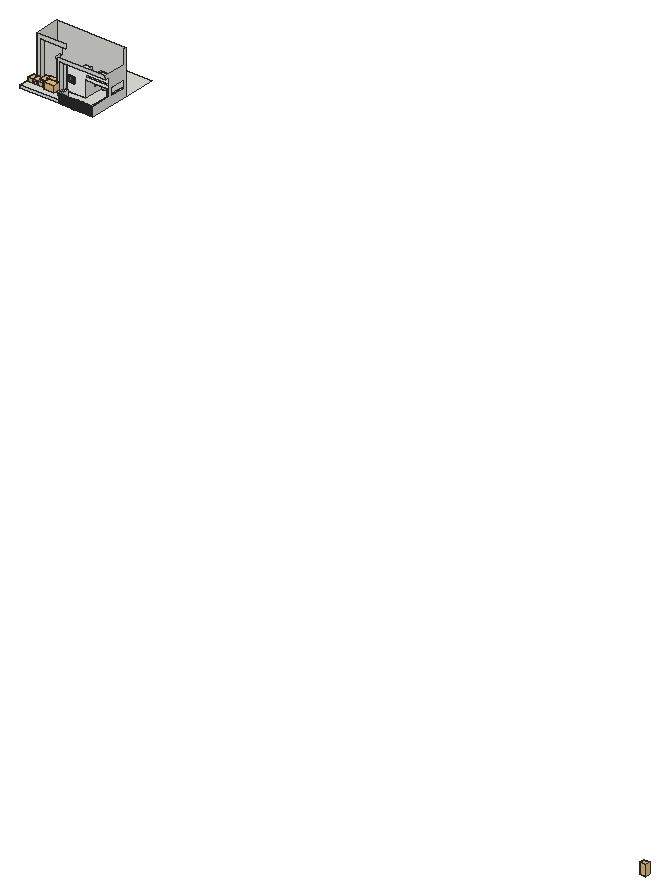
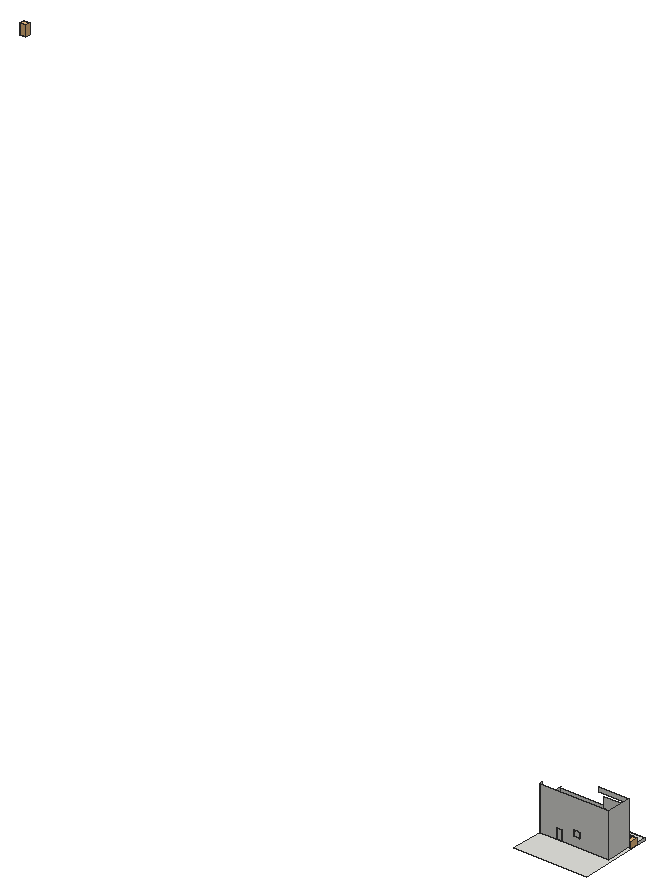
# SketchUp Ruby script. Lengths in inches.
U = 1.inch
M = Sketchup.active_model
def pt(a) = Geom::Point3d.new(a.map { |v| v * U })
def face(e, loops, mat)
  f = e.add_face(loops[0].map { |a| pt(a) })
  loops[1..].each { |l| e.add_face(l.map { |a| pt(a) }).erase! }
  f.material = f.back_material = mat if mat
  f
end
# faces: each face lists its corners as indices into pts; further lists are holes
def faces(e, pts, list, mat = nil) = list.each { |f| face(e, (f[0].is_a?(Array) ? f : [f]).map { |l| l.map { |i| pts[i] } }, mat) }
# xy, xz, yz: faces in a plane at the given z, y or x. An outline is a flat list of corners, or four numbers for a rectangle; further outlines are holes
def ring(l) = l.size == 4 ? [[l[0], l[1]], [l[2], l[1]], [l[2], l[3]], [l[0], l[3]]] : l.each_slice(2).to_a
def flat(e, list, mat, &to3) = list.each { |f| face(e, (f[0].is_a?(Array) ? f : [f]).map { |l| ring(l).map { |u, v| to3.(u, v) } }, mat) }
def xy(e, z, list, mat = nil) = flat(e, list, mat) { |x, y| [x, y, z] }
def xz(e, y, list, mat = nil) = flat(e, list, mat) { |x, z| [x, y, z] }
def yz(e, x, list, mat = nil) = flat(e, list, mat) { |y, z| [x, y, z] }
def lines(e, pts, list) = list.each { |a, b| e.add_line(pt(pts[a]), pt(pts[b])) }
# prism: a flat outline (further loops are holes) pulled along v
def prism(e, loops, v, mat = nil)
  f = face(e, loops, mat); d = Geom::Vector3d.new(v.map { |x| x * U })
  f.pushpull(f.normal.samedirection?(d) ? d.length : -d.length)
end
def box(e, o, s, mat = nil) = prism(e, [[o, [o[0] + s[0], o[1], o[2]], [o[0] + s[0], o[1] + s[1], o[2]], [o[0], o[1] + s[1], o[2]]]], [0, 0, s[2]], mat)
def at(x, y, z, deg = 0) = Geom::Transformation.translation(pt([x, y, z])) * Geom::Transformation.rotation(ORIGIN, Z_AXIS, deg.degrees)
def axes(o, x, y, z) = Geom::Transformation.new([*x, 0, *y, 0, *z, 0, *pt(o).to_a, 1])
def part(name) = M.definitions.add(name)
# library, detail: a bought-in or finely detailed component or shape, given as its bounding box
def library(name, o, s) = part(name).tap { |d| box(d.entities, o, s) }
def detail(e, o, s) = box(e.add_group.entities, o, s)
def put(e, d, t, mat = nil) = e.add_instance(d, t).tap { |i| i.material = mat if mat }
def group(e, t, mat = nil) = e.add_group.tap { |g| g.transformation = t; g.material = mat if mat }.entities
root = M.entities
M.materials.add("[0131_Silver]").color = [192, 192, 192]
M.materials.add("[Color M00]").color = [255, 255, 255]
M.materials.add("[Translucent Glass Gray]").color = [128, 128, 128]
M.materials["[Translucent Glass Gray]"].alpha = 0.5
M.materials.add("[Wood Floor]").color = [155, 105, 61]
M.materials.add("efeu2").color = [43, 57, 29]
c1 = library("Broadleaf plant",[0,0,0],[149.19,166.1,98.1875])
c2 = library("N_Plant_4",[-12.12,-0.17,0],[15.33,15.33,4.43])
c3 = library("door by lz",[5.91,-4.92,0],[35.43,6.61,78.74])
c4 = part("Gate frame")
xy(c4.entities,0,[[[0,0,66,72],[3,3,48,69],[51,3,63,69]]])
xy(c4.entities,0.5,[[3,3,48,69]])
xy(c4.entities,1.5,[[3,3,48,11.25],[3,11.25,48,19.5],[3,19.5,48,27.75],[3,27.75,48,36],[3,36,48,44.25],
  [3,44.25,48,52.5],[3,52.5,48,60.75],[3,60.75,48,69]])
xy(c4.entities,2,[[[0,0,66,72],[3,3,48,69],[51,3,63,69]]])
xz(c4.entities,0,[[0,0,51,2],[51,0,66,2]])
xz(c4.entities,3,[[3,0,27,0.5],[27,0,48,0.5],[51,0,63,2],[3,1.5,48,2]])
xz(c4.entities,69,[[3,0,48,0.5],[51,0,63,2],[3,1.5,48,2]])
xz(c4.entities,72,[[0,0,66,2]])
yz(c4.entities,0,[[0,0,72,2]])
yz(c4.entities,3,[[3,0,69,0.5],[3,1.5,69,2]])
yz(c4.entities,48,[[3,0,69,0.5],[3,1.5,69,2]])
yz(c4.entities,51,[[3,0,69,2]])
yz(c4.entities,63,[[3,0,69,2]])
yz(c4.entities,66,[[0,0,72,2]])
c5 = part("Horizontal gate bar")
box(c5.entities,[0,0,0],[12,1,1])
c6 = part("Slatted gate insert")
put(c6.entities,c5,at(3,0.5,22.5))
put(c6.entities,c5,at(3,0.5,26.5))
put(c6.entities,c5,at(3,0.5,28.5))
put(c6.entities,c5,at(3,0.5,4.5))
put(c6.entities,c5,at(3,0.5,2.5))
put(c6.entities,c5,at(3,0.5,54.5))
put(c6.entities,c5,at(3,0.5,56.5))
put(c6.entities,c5,at(3,0.5,24.5))
put(c6.entities,c5,at(3,0.5,20.5))
put(c6.entities,c5,at(3,0.5,34.5))
put(c6.entities,c5,at(3,0.5,6.5))
put(c6.entities,c5,at(3,0.5,42.5))
put(c6.entities,c5,at(3,0.5,0.5))
put(c6.entities,c5,at(3,0.5,10.5))
put(c6.entities,c5,at(3,0.5,16.5))
put(c6.entities,c5,at(3,0.5,18.5))
put(c6.entities,c5,at(3,0.5,58.5))
put(c6.entities,c5,at(3,0.5,40.5))
put(c6.entities,c5,at(3,0.5,60.5))
put(c6.entities,c5,at(3,0.5,36.5))
put(c6.entities,c5,at(3,0.5,38.5))
put(c6.entities,c5,at(3,0.5,32.5))
put(c6.entities,c5,at(3,0.5,8.5))
put(c6.entities,c5,at(3,0.5,64.5))
put(c6.entities,c5,at(3,0.5,12.5))
put(c6.entities,c5,at(3,0.5,44.5))
put(c6.entities,c5,at(3,0.5,46.5))
put(c6.entities,c5,at(3,0.5,52.5))
put(c6.entities,c5,at(3,0.5,48.5))
put(c6.entities,c5,at(3,0.5,50.5))
put(c6.entities,c5,at(3,0.5,62.5))
put(c6.entities,c5,at(3,0.5,14.5))
put(c6.entities,c5,at(3,0.5,30.5))
c7 = part("Gate panel slat")
xy(c7.entities,0.25,[[0.25,0,44.75,0.15]])
xy(c7.entities,8,[[0.25,0,44.75,0.15]])
xz(c7.entities,0,[[0.25,0.25,44.75,8]])
xz(c7.entities,0.15,[[[0,0,45,8.25],[0.25,0.25,44.75,8]]])
yz(c7.entities,0.25,[[0,0.25,0.15,8]])
yz(c7.entities,44.75,[[0,0.25,0.15,8]])
p = [[0,0.15,0],[0.25,0,0.25],[44.75,0,0.25],[45,0.15,0],[0,0.15,8.25],[0.25,0,8],
  [44.75,0,8],[45,0.15,8.25]]
faces(c7.entities,p,[[0,1,2,3],[4,5,1,0],[3,2,6,7],[5,4,7,6]])
c8 = part("Gate infill panel")
put(c8.entities,c7,at(0,0,24.75))
put(c8.entities,c7,at(0,0,57.75))
put(c8.entities,c7,at(0,0,49.5))
put(c8.entities,c7,at(0,0,41.25))
put(c8.entities,c7,at(0,0,33))
put(c8.entities,c7,axes([0,1.3,49.5],[1,0,0],[0,-1,0],[0,0,1]))
put(c8.entities,c7,at(0,0,16.5))
put(c8.entities,c7,at(0,0,8.25))
put(c8.entities,c7,axes([0,1.3,24.75],[1,0,0],[0,-1,0],[0,0,1]))
put(c8.entities,c7,at(0,0,0))
put(c8.entities,c7,axes([0,1.3,57.75],[1,0,0],[0,-1,0],[0,0,1]))
put(c8.entities,c7,axes([0,1.3,41.25],[1,0,0],[0,-1,0],[0,0,1]))
put(c8.entities,c7,axes([0,1.3,33],[1,0,0],[0,-1,0],[0,0,1]))
put(c8.entities,c7,axes([0,1.3,16.5],[1,0,0],[0,-1,0],[0,0,1]))
put(c8.entities,c7,axes([0,1.3,8.25],[1,0,0],[0,-1,0],[0,0,1]))
put(c8.entities,c7,axes([0,1.3,0],[1,0,0],[0,-1,0],[0,0,1]))
c9 = part("Entrance gate leaf")
put(c9.entities,c4,axes([0,2,0],[1,0,0],[0,0,1],[0,-1,0]),"[0131_Silver]")
put(c9.entities,c6,at(48,0,3),"[0131_Silver]")
put(c9.entities,c8,at(3,0.35,3))
c10 = part("Gate pull handle")
prism(c10.entities,[[[0.35,0,3.8],[0.35,0,3],[0.35,-1.5,3],[0.35,-1.5,51],[0.35,0,51],[0.35,0,50.2],[0.35,-1,50.2],[0.35,-1,3.8]]],[0.8,0,0])
c11 = part("gate1")
g1 = group(c11.entities,at(123.625,43.75,0))
put(g1,c9,at(0,1.5,0))
put(g1,c10,at(67.25,1.5,9),"[0131_Silver]")
put(g1,c10,at(63.75,1.5,9),"[0131_Silver]")
put(g1,c9,axes([132.5,1.5,0],[-1,0,0],[0,1,0],[0,0,1]))
c12 = part("window full")
xy(c12.entities,0,[[0,0,14.17,66.54]])
xy(c12.entities,2.26,[[12.2,2.26,14.17,64.28]],"[Wood Floor]")
xy(c12.entities,2.36,[[0,2.36,1.97,64.17]],"[Wood Floor]")
xy(c12.entities,3.74,[[11.42,3.74,12.2,32.875],[11.42,33.66,12.2,62.79]],"[Wood Floor]")
xy(c12.entities,3.9375,[[1.97,3.9375,2.76,32.77],[1.97,33.76,2.76,62.6]],"[Wood Floor]")
xy(c12.entities,4.18,[[2.76,4.18,7.09,32.09],[7.09,4.18,11.42,32.09],[2.76,34.45,7.09,62.35],[7.09,34.45,11.42,62.35]],"[Wood Floor]")
xy(c12.entities,69.83,[[2.76,4.18,7.09,32.09],[7.09,32.09,11.42,34.45],[2.76,34.45,7.09,62.35]])
xy(c12.entities,69.83,[[7.09,4.18,11.42,32.09],[7.09,34.45,11.42,62.35]],"[Wood Floor]")
xy(c12.entities,70.08,[[1.97,3.9375,2.76,32.77],[1.97,33.76,2.76,62.6]])
xy(c12.entities,70.27,[[11.42,32.875,12.2,33.66]])
xy(c12.entities,70.27,[[11.42,3.74,12.2,32.875],[11.42,33.66,12.2,62.79]],"[Wood Floor]")
xy(c12.entities,71.65,[[0,2.36,1.97,64.17]])
xy(c12.entities,71.76,[[12.2,2.26,14.17,64.28]],"[Wood Floor]")
xy(c12.entities,74.02,[[0,0,14.17,66.54]],"[Wood Floor]")
xz(c12.entities,0,[[0,0,14.17,74.02]],"[Wood Floor]")
xz(c12.entities,2.26,[[12.2,2.26,14.17,71.76]],"[Wood Floor]")
xz(c12.entities,2.36,[[0,2.36,1.97,71.65]],"[Wood Floor]")
xz(c12.entities,3.74,[[11.42,3.74,12.2,70.27]],"[Wood Floor]")
xz(c12.entities,3.9375,[[1.97,3.9375,2.76,70.08]],"[Wood Floor]")
xz(c12.entities,4.18,[[2.76,4.18,7.09,69.83],[7.09,4.18,11.42,69.83]],"[Wood Floor]")
xz(c12.entities,32.09,[[2.76,4.18,11.42,69.83]],"[Wood Floor]")
xz(c12.entities,32.77,[[1.97,3.9375,2.76,70.08]],"[Wood Floor]")
xz(c12.entities,32.875,[[11.42,3.74,12.2,70.27]],"[Wood Floor]")
xz(c12.entities,33.66,[[11.42,3.74,12.2,47.88],[11.42,47.88,12.2,70.27]],"[Wood Floor]")
xz(c12.entities,33.76,[[1.97,3.9375,2.76,70.08]],"[Wood Floor]")
xz(c12.entities,34.45,[[2.76,4.18,11.42,69.83]],"[Wood Floor]")
xz(c12.entities,62.35,[[2.76,4.18,7.09,69.83],[7.09,4.18,11.42,69.83]],"[Wood Floor]")
xz(c12.entities,62.6,[[1.97,3.9375,2.76,70.08]],"[Wood Floor]")
xz(c12.entities,62.79,[[11.42,3.74,12.2,70.27]],"[Wood Floor]")
xz(c12.entities,64.17,[[0,2.36,1.97,71.65]],"[Wood Floor]")
xz(c12.entities,64.28,[[12.2,2.26,14.17,71.76]],"[Wood Floor]")
xz(c12.entities,66.54,[[0,0,14.17,74.02]],"[Wood Floor]")
yz(c12.entities,0,[[[0,0,66.54,74.02],[2.36,2.36,64.17,71.65]]],"[Wood Floor]")
yz(c12.entities,1.97,[[[2.36,2.36,64.17,71.65],[33.76,3.9375,62.6,70.08],[3.9375,3.9375,32.77,70.08]]],"[Wood Floor]")
yz(c12.entities,2.76,[[32.77,3.9375,33.76,4.18],[32.77,4.18,33.76,69.83],[32.77,69.83,33.76,70.08]])
yz(c12.entities,2.76,[[[3.9375,3.9375,32.77,70.08],[4.18,4.18,32.09,69.83]],[[33.76,3.9375,62.6,70.08],[34.45,4.18,62.35,69.83]]],"[Wood Floor]")
yz(c12.entities,7.09,[[4.18,4.18,62.35,69.83]],"[Translucent Glass Gray]")
yz(c12.entities,11.42,[[32.875,69.83,33.66,70.27]])
yz(c12.entities,11.42,[[[3.74,3.74,32.875,70.27],[4.18,4.18,32.09,69.83]],[[33.66,3.74,62.79,70.27],[34.45,4.18,62.35,69.83]]],"[Wood Floor]")
yz(c12.entities,12.2,[[[2.26,2.26,64.28,71.76],[3.74,3.74,32.875,70.27],[33.66,3.74,62.79,70.27]]],"[Wood Floor]")
yz(c12.entities,14.17,[[[0,0,66.54,74.02],[2.26,2.26,64.28,71.76]]],"[Wood Floor]")
p = [[11.42,32.875,70.27],[11.42,32.875,70.28]]
lines(c12.entities,p,[[0,1]])
c13 = library("climbing plant",[8874.76,-5589.78,-33.625],[50.13,38.07,87.16])
c14 = part("ivyleaf_10")
p = [[0,0.5,-0.03],[-0.0625,2.02,-0.43],[-0.19,2.01,-0.46],[-0.54,1.05,-0.29],[-0.52,0.625,-0.18],[-0.83,0.76,-0.28],
  [-1.16,0.64,-0.33],[-1.15,0.33,-0.24],[-0.77,-0.39,0.02],[-0.3,-0.51,0.16],[0.04,-0.48,0.23],[-0.02,2.01,-0.4375],
  [-0.06,2.01,-0.43],[0.04,-0.49,0.23],[0.67,-0.49,0.14],[1.38,0.36,-0.2],[1.375,0.51,-0.24],[0.81,0.65,-0.19],
  [0.62,0.59,-0.15],[0.6,1.09,-0.28],[0.5,1.23,-0.31]]
faces(c14.entities,p,[[0,1,2,3,4,5,6,7,8,9,10],[11,12,0,13,14,15,16,17,18,19,20]],"efeu2")
xy(root,0,[[0,7.0625,315.8125,80.4375],[336.86,7.0625,583.09,7.0625,583.09,321.4375,460.26,321.4375,460.26,345.4375,412.26,345.4375,412.26,172.6875,255.63,172.6875,255.63,166.9375,222.91,166.9375,222.91,139.625,196.34,139.625,196.34,172.6875,63.85,172.6875,63.85,139.625,29.66,139.625,29.66,345.4375,600,345.4375,600,607.0625,0,607.0625,0,80.4375,315.8125,80.4375,315.8125,81.3125,336.86,81.3125],[583.09,7.0625,600,81.3125],[583.09,81.3125,600,172.6875],[29.66,139.625,29.66,345.4375,412.26,345.4375,412.26,172.6875,255.63,172.6875,255.63,166.9375,222.91,166.9375,222.91,139.625,196.34,139.625,196.34,172.6875,63.85,172.6875,63.85,139.625],
  [583.09,172.6875,583.09,321.4375,460.26,321.4375,460.26,345.4375,600,345.4375,600,172.6875]])
xy(root,23.375,[[0,7.0625,315.8125,80.4375]])
xy(root,65.15,[[583.09,0,600,7.0625]])
xy(root,65.68,[[315.8125,3.1875,336.86,7.0625]])
xy(root,70.625,[[583.09,0,600,172.6875],[315.8125,3.1875,336.86,81.3125],[583.09,191.6,600,321.4375]])
xy(root,71.7,[[267.6,172.6875,315.6,345.4375]])
xy(root,84,[[412.26,321.4375,460.26,345.4375]])
xy(root,119.7,[[267.6,172.6875,315.6,345.4375]])
xy(root,129.8125,[[412.26,172.6875,583.09,321.4375],[583.09,191.6,600,321.4375]])
xz(root,0,[[583.09,65.15,600,70.625]])
xz(root,3.1875,[[315.8125,65.68,336.86,70.625]])
xz(root,7.0625,[[0,0,315.8125,23.375],[315.8125,0,336.86,65.68],[583.09,0,600,65.15]])
xz(root,80.4375,[[0,0,315.8125,23.375]])
xz(root,81.3125,[[315.8125,0,336.86,70.625]])
xz(root,139.625,[[29.66,0,63.85,0,63.85,328.1875,270.19,328.1875,270.19,360,29.66,360],[196.34,0,222.91,0,222.91,212.04,600,212.04,600,240.74,196.34,240.74]])
xz(root,166.9375,[[222.91,0,255.63,212.04]])
xz(root,172.6875,[[63.85,0,196.34,0,196.34,244.35,209.625,244.35,209.625,328.1875,63.85,328.1875]])
xz(root,172.6875,[[[255.63,0,255.63,212.04,600,212.04,600,171.1,412.26,171.1,412.26,154.12,600,154.12,600,70.625,583.09,70.625,583.09,129.8125,412.26,129.8125,412.26,0],[267.6,71.7,315.6,119.7]]],"[Color M00]")
xz(root,191.6,[[583.09,70.625,600,129.8125]])
xz(root,321.4375,[[460.26,0,583.09,0,583.09,70.625,600,70.625,600,129.8125,412.26,129.8125,412.26,84,460.26,84]])
xz(root,345.4375,[[[29.66,0,29.66,360,600,360,600,0,460.26,0,460.26,84,412.26,84,412.26,0],[267.6,71.7,315.6,119.7]],[412.26,0,460.26,84],[267.6,71.7,315.6,119.7]])
yz(root,0,[[7.0625,0,80.4375,23.375]])
yz(root,29.66,[[139.625,0,345.4375,360]])
yz(root,63.85,[[139.625,0,172.6875,328.1875]])
yz(root,196.34,[[139.625,0,139.625,240.74,130,240.74,130,244.35,172.6875,244.35,172.6875,0]])
yz(root,222.91,[[139.625,0,166.9375,212.04]])
yz(root,255.63,[[166.9375,0,172.6875,212.04]])
yz(root,267.6,[[172.6875,71.7,345.4375,119.7]])
yz(root,315.6,[[172.6875,71.7,345.4375,119.7]])
yz(root,315.8125,[[7.0625,0,80.4375,23.375],[80.4375,0,81.3125,23.375],[7.0625,23.375,7.0625,65.68,3.1875,65.68,3.1875,70.625,80.4375,70.625,80.4375,23.375],[80.4375,23.375,81.3125,70.625]])
yz(root,336.86,[[7.0625,0,81.3125,0,81.3125,70.625,3.1875,70.625,3.1875,65.68,7.0625,65.68]])
yz(root,412.26,[[172.6875,0,345.4375,0,345.4375,84,321.4375,84,321.4375,117.76,172.6875,129.8125],[321.4375,117.76,321.4375,129.8125,172.6875,129.8125]])
yz(root,460.26,[[321.4375,0,345.4375,84]])
yz(root,583.09,[[7.0625,0,7.0625,65.15,0,65.15,0,70.625,172.6875,70.625,172.6875,129.8125,191.6,129.8125,191.6,70.625,321.4375,70.625,321.4375,0]])
yz(root,600,[[7.0625,0,345.4375,0,345.4375,360,319,360,319,244.35,130,244.35,130,240.74,139.625,240.74,139.625,212.04,172.6875,212.04,172.6875,129.8125,321.4375,129.8125,321.4375,70.625,191.6,70.625,191.6,129.8125,172.6875,129.8125,172.6875,70.625,0,70.625,0,65.15,7.0625,65.15]])
p = [[412.26,321.4375,117.76],[412.26,344.1875,115.92],[412.26,321.4375,129.8125],[412.26,344.1875,129.8125],[315.8125,81.3125,75.5],[315.8125,80.4375,75.5],
  [315.8125,7.0625,75.5],[315.8125,7.0625,75.8125],[315.8125,80.4375,75.8125],[332.61,7.0625,75.5],[332.61,7.0625,75.8125]]
lines(root,p,[[0,1],[2,3],[4,5],[6,7],[5,8],[9,10]])
put(root,c1,axes([123.46,132.97,-11.69],[0.55836,0,0],[0,0.396,0],[0,0,0.74781]))
put(root,c2,axes([155.86,80.09,-1.59],[5.46099,0,0],[0,3.78,0],[0,0,11.75209]))
put(root,c2,axes([72.99,80.09,-1.59],[5.46099,0,0],[0,3.78,0],[0,0,11.75209]))
put(root,c2,axes([110.36,80.09,-1.59],[5.46099,0,0],[0,3.78,0],[0,0,11.75209]))
put(root,c3,axes([403.66,324.07,0],[1.369,0,0],[0,-1.55488,0],[0,0,1.0668]))
put(root,c11,axes([106.65,-38.1875,0],[1.86484,0,0],[0,1,0],[0,0,1]))
put(root,c1,axes([86.08,103.09,12.29],[0.396,0,0],[0,0.396,0],[0,0,0.4733]))
put(root,c2,axes([216.73,59.6875,23.375],[5.46099,0,0],[0,3.78,0],[0,0,11.75209]))
put(root,c12,axes([266.09,182.18,70.1875],[0,-0.67,0],[0.74416,0,0],[0,0,0.67]))
put(root,c13,at(762.05,-85.8125,132.37))
put(root,c14,axes([515.27,136.46,139.07],[-0.1022,0.53332,-0.33609],[0.06573,-0.32961,-0.54301],[-0.62695,-0.12149,-0.00215]))
put(root,c14,axes([585.06,128.8,139.52],[0.29691,-0.31047,-0.60423],[-0.41367,0.44043,-0.42957],[0.53885,0.50919,0.00315]))
put(root,c14,axes([585.27,128.82,140.01],[-0.61261,0.1438,-0.24217],[0.23254,-0.06883,-0.62913],[-0.1589,-0.65514,0.01295]))
put(root,c14,axes([586.2,127.32,140.4],[0.10431,-0.29788,0.60644],[0.16756,-0.58305,-0.31522],[0.65454,0.19673,-0.01595]))
